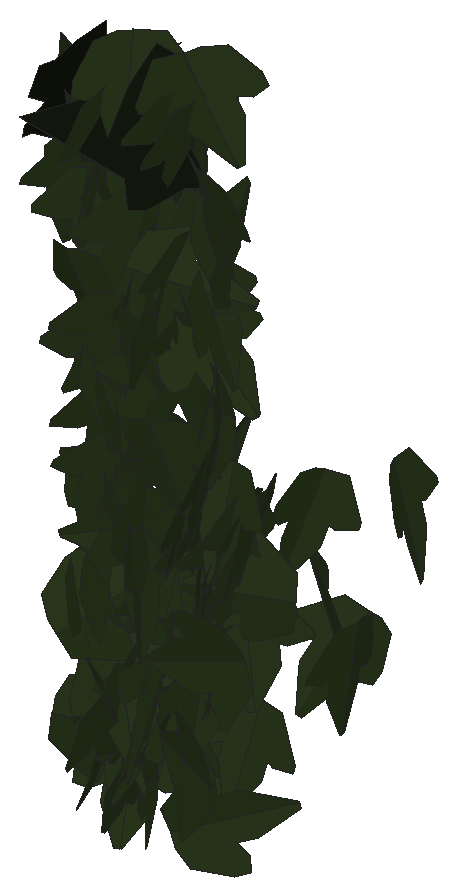
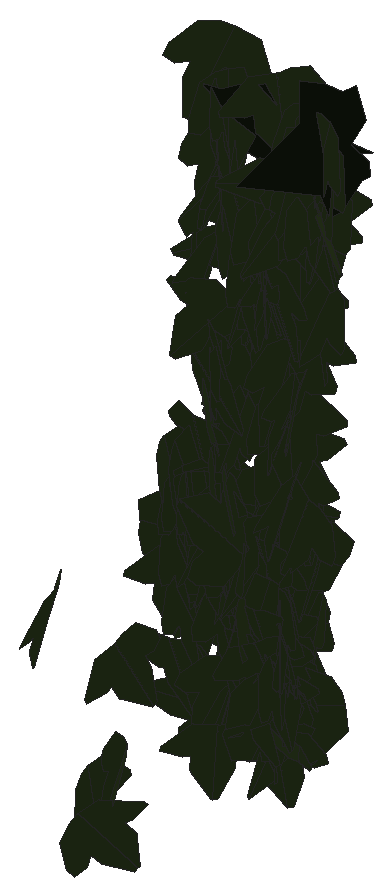
# SketchUp Ruby script. Lengths in inches.
U = 1.inch
M = Sketchup.active_model
def pt(a) = Geom::Point3d.new(a.map { |v| v * U })
def face(e, loops, mat)
  f = e.add_face(loops[0].map { |a| pt(a) })
  loops[1..].each { |l| e.add_face(l.map { |a| pt(a) }).erase! }
  f.material = f.back_material = mat if mat
  f
end
# faces: each face lists its corners as indices into pts; further lists are holes
def faces(e, pts, list, mat = nil) = list.each { |f| face(e, (f[0].is_a?(Array) ? f : [f]).map { |l| l.map { |i| pts[i] } }, mat) }
# xy, xz, yz: faces in a plane at the given z, y or x. An outline is a flat list of corners, or four numbers for a rectangle; further outlines are holes
def ring(l) = l.size == 4 ? [[l[0], l[1]], [l[2], l[1]], [l[2], l[3]], [l[0], l[3]]] : l.each_slice(2).to_a
def flat(e, list, mat, &to3) = list.each { |f| face(e, (f[0].is_a?(Array) ? f : [f]).map { |l| ring(l).map { |u, v| to3.(u, v) } }, mat) }
def xy(e, z, list, mat = nil) = flat(e, list, mat) { |x, y| [x, y, z] }
def xz(e, y, list, mat = nil) = flat(e, list, mat) { |x, z| [x, y, z] }
def yz(e, x, list, mat = nil) = flat(e, list, mat) { |y, z| [x, y, z] }
def lines(e, pts, list) = list.each { |a, b| e.add_line(pt(pts[a]), pt(pts[b])) }
# prism: a flat outline (further loops are holes) pulled along v
def prism(e, loops, v, mat = nil)
  f = face(e, loops, mat); d = Geom::Vector3d.new(v.map { |x| x * U })
  f.pushpull(f.normal.samedirection?(d) ? d.length : -d.length)
end
def box(e, o, s, mat = nil) = prism(e, [[o, [o[0] + s[0], o[1], o[2]], [o[0] + s[0], o[1] + s[1], o[2]], [o[0], o[1] + s[1], o[2]]]], [0, 0, s[2]], mat)
def at(x, y, z, deg = 0) = Geom::Transformation.translation(pt([x, y, z])) * Geom::Transformation.rotation(ORIGIN, Z_AXIS, deg.degrees)
def axes(o, x, y, z) = Geom::Transformation.new([*x, 0, *y, 0, *z, 0, *pt(o).to_a, 1])
def part(name) = M.definitions.add(name)
# library, detail: a bought-in or finely detailed component or shape, given as its bounding box
def library(name, o, s) = part(name).tap { |d| box(d.entities, o, s) }
def detail(e, o, s) = box(e.add_group.entities, o, s)
def put(e, d, t, mat = nil) = e.add_instance(d, t).tap { |i| i.material = mat if mat }
def group(e, t, mat = nil) = e.add_group.tap { |g| g.transformation = t; g.material = mat if mat }.entities
root = M.entities
M.materials.add("efeu1").color = [18, 25, 13]
M.materials.add("efeu2").color = [43, 57, 29]
c1 = part("ivyleaf_10")
p = [[0,0.5,-0.03],[-0.0625,2.02,-0.43],[-0.19,2.01,-0.46],[-0.54,1.05,-0.29],[-0.52,0.625,-0.18],[-0.83,0.76,-0.28],
  [-1.16,0.64,-0.33],[-1.15,0.33,-0.24],[-0.77,-0.39,0.02],[-0.3,-0.51,0.16],[0.04,-0.48,0.23],[-0.02,2.01,-0.4375],
  [-0.06,2.01,-0.43],[0.04,-0.49,0.23],[0.67,-0.49,0.14],[1.38,0.36,-0.2],[1.375,0.51,-0.24],[0.81,0.65,-0.19],
  [0.62,0.59,-0.15],[0.6,1.09,-0.28],[0.5,1.23,-0.31]]
faces(c1.entities,p,[[0,1,2,3,4,5,6,7,8,9,10],[11,12,0,13,14,15,16,17,18,19,20]],"efeu2")
c2 = part("ivyleaf_9")
p = [[1.54,2.16,1.25],[1.36,2.04,1.19],[-0.21,0.99,0.68],[-0.71,1.11,0.82],[-0.85,0.86,0.67],[-0.8,0.17,0.21],
  [-0.9,-0.01,0.1],[-0.67,-0.16,-0.02],[-0.08,-0.08,-0.05],[-0.03,-0.6,-0.4],[0.65,-0.88,-0.66],[0.83,-0.6,-0.49],
  [1.29,-0.42,-0.43],[1.8125,-0.07,-0.26],[1.21,0.44,0.15]]
faces(c2.entities,p,[[0,1,2,3,4,5,6,7,8,9,10,11,12,13,14]],"efeu1")
put(root,c1,axes([521.63,138.375,173.66],[0.03642,-0.63597,0.0421],[0.01639,-0.04122,-0.63686],[0.63715,0.03741,0.01397]))
put(root,c1,axes([521.68,137.33,181.72],[-0.16201,-0.67993,0.11129],[0.00026,-0.11439,-0.69846],[0.68898,-0.15984,0.02643]))
put(root,c1,axes([521.59,137.31,183],[-0.63085,0.3128,-0.09955],[0.04645,-0.12842,-0.69791],[-0.32495,-0.62562,0.09349]))
put(root,c1,axes([521.7,137.19,181.875],[-0.58468,0.38831,0.11251],[-0.11108,0.0359,-0.70119],[-0.38872,-0.59433,0.03116]))
put(root,c1,axes([521.73,137.81,173.7],[0.04033,-0.60534,-0.30444],[-0.00149,0.3049,-0.60645],[0.67758,0.0367,0.01678]))
put(root,c1,axes([521.33,137.39,181.05],[0.34543,-0.39762,-0.46848],[0.32054,-0.34191,0.52654],[-0.52424,-0.47106,0.01326]))
put(root,c2,axes([521.49,136.8,182.72],[0.24079,0.34365,0.64076],[0.3954,0.50457,-0.41919],[-0.61019,0.46256,-0.01878]))
put(root,c1,axes([521.68,138.15,174.76],[0.45192,-0.45158,-0.15955],[0.02127,0.23808,-0.61358],[0.47847,0.41594,0.17798]))
put(root,c1,axes([521.73,137.08,182.4375],[-0.65958,0.28506,-0.00532],[0.00194,-0.00894,-0.71851],[-0.28511,-0.65954,0.00744]))
put(root,c1,axes([521.42,137.88,176.49],[0.59836,-0.14425,0.27817],[0.30389,0.12093,-0.59097],[0.07641,0.64868,0.17203]))
put(root,c1,axes([521.66,138.17,174.29],[0.41426,-0.50056,0.10032],[0.10441,-0.04339,-0.64765],[0.49972,0.42402,0.05216]))
put(root,c1,axes([521.6875,137.17,180],[-0.63481,0.21978,-0.15697],[0.14667,-0.05616,-0.67176],[-0.22678,-0.65151,0.00495]))
put(root,c1,axes([522.03,137.49,176.72],[-0.62326,-0.0477,0.26578],[-0.26115,-0.0635,-0.6238],[0.06865,-0.67458,0.03993]))
put(root,c1,axes([521.92,138.41,173.25],[-0.3203,-0.53428,0.14995],[-0.00408,-0.17086,-0.61751],[0.55491,-0.30965,0.082]))
put(root,c1,axes([521.67,137.84,172.2],[-0.08853,-0.45137,-0.44245],[0.13261,-0.45009,0.43263],[-0.61799,-0.03192,0.15622]))
put(root,c1,axes([521.64,137.39,181.92],[-0.37113,-0.35946,-0.48251],[0.37331,0.30704,-0.51587],[0.47187,-0.52562,0.02863]))
put(root,c1,axes([521.93,138.38,172.29],[0.24532,0.56679,0.17941],[-0.06142,-0.16889,0.61752],[0.59133,-0.25268,-0.0103]))
put(root,c1,axes([521.98,136.99,174.07],[-0.51698,0.35185,0.17256],[-0.13825,0.10353,-0.62531],[-0.36668,-0.5351,-0.00752]))
put(root,c1,axes([521.83,137.77,178.42],[-0.43298,0.49382,-0.19017],[0.0645,-0.19463,-0.65226],[-0.52522,-0.43099,0.07667]))
put(root,c1,axes([521.4,137.54,172.83],[-0.12186,-0.03802,-0.69789],[0.68926,0.11084,-0.12639],[0.1158,-0.69972,0.0179]))
put(root,c1,axes([521.85,137.09,175.36],[-0.12313,0.68542,0.03123],[-0.0099,0.02995,-0.69638],[-0.68606,-0.12345,0.00444]))
put(root,c1,axes([522.04,137.58,177.97],[-0.34,-0.5928,0.00312],[-0.01009,0.0022,-0.68331],[0.59272,-0.34,-0.00985]))
put(root,c1,axes([521.95,138.38,173.95],[0.50097,0.35528,-0.1951],[-0.15047,-0.125,-0.614],[-0.37636,0.52288,-0.01422]))
put(root,c1,axes([521.88,138.03,172.17],[0.57312,0.28141,-0.0286],[-0.0251,-0.01377,-0.63848],[-0.28174,0.57366,-0.00129]))
put(root,c1,axes([521.9,137.78,176.71],[-0.18245,0.65594,0.01519],[0.0107,0.01874,-0.68067],[-0.65603,-0.18212,-0.01533]))
put(root,c1,axes([522.03,138.22,174.35],[0.60863,-0.1362,-0.15762],[-0.13614,0.10836,-0.61931],[0.15767,0.6193,0.0737]))
put(root,c1,axes([522.15,137.48,177.14],[-0.26854,-0.56151,0.25077],[-0.06831,-0.24471,-0.62109],[0.61116,-0.27407,0.04077]))
put(root,c1,axes([522.04,137.43,178.32],[-0.19363,0.62062,0.25663],[-0.09885,0.23784,-0.64975],[-0.66427,-0.2163,0.02188]))
put(root,c1,axes([521.99,137.36,181.68],[-0.02174,-0.32316,-0.72112],[0.15706,0.70523,-0.32077],[0.77445,-0.1521,0.04481]))
put(root,c1,axes([522.08,137.24,181.32],[-0.5316,-0.47405,0.02236],[0.08346,-0.12644,-0.69633],[0.46718,-0.51683,0.14984]))
put(root,c1,axes([522.2,137.12,179.11],[-0.61368,-0.27764,0.07523],[-0.03254,-0.10912,-0.66812],[0.28581,-0.60857,0.08547]))
put(root,c1,axes([522.12,137.625,172.21],[-0.02606,-0.38595,-0.51186],[0.04871,0.50961,-0.38673],[0.63921,-0.05457,0.0086]))
put(root,c1,axes([522.07,137.51,178.86],[-0.26527,-0.5787,-0.25013],[0.15361,0.20386,-0.63456],[0.61144,-0.30228,0.0509]))
put(root,c1,axes([522.3,142.29,172.375],[-0.32073,-0.37581,0.43332],[-0.02427,-0.48712,-0.44044],[0.57307,-0.23096,0.22386]))
put(root,c1,axes([522.25,138.17,172.9],[-0.19878,0.22652,0.58226],[0.02919,-0.60699,0.2461],[0.62408,0.10054,0.17395]))
put(root,c1,axes([522.22,138.06,174.73],[-0.65389,0.00582,-0.06624],[0.06629,0.00603,-0.65389],[-0.00518,-0.65721,-0.00659]))
put(root,c1,axes([521.8,137.38,182.13],[-0.01198,-0.03667,0.70751],[0.48021,0.51984,0.03507],[-0.52088,0.48009,0.01606]))
put(root,c1,axes([522.26,137,182.88],[-0.02378,-0.65358,-0.27372],[0.06735,0.27055,-0.65186],[0.70537,-0.04786,0.05301]))
put(root,c1,axes([522.22,141.71,173.38],[-0.44013,0.46308,-0.00992],[0.00995,-0.00423,-0.63886],[-0.46308,-0.44023,-0.00429]))
put(root,c1,axes([522.25,136.91,175.63],[-0.10043,0.55451,0.38958],[-0.09847,0.37772,-0.56301],[-0.67049,-0.13853,0.02433]))
put(root,c1,axes([522.7,137.67,176.16],[0.09478,0.07272,-0.66694],[-0.62373,-0.23852,-0.11465],[-0.24708,0.63,0.03358]))
put(root,c1,axes([522.03,137.92,173.1],[0.5933,0.06495,0.23202],[0.23022,0.02907,-0.59684],[-0.07106,0.63639,0.00358]))
put(root,c1,axes([522.24,137.56,173.14],[0.62736,-0.16316,0.01158],[0.01079,-0.00451,-0.64823],[0.16322,0.62745,-0.00165]))
put(root,c1,axes([522.36,137.55,180.3],[0.59763,-0.33867,-0.11277],[-0.08526,0.07812,-0.68645],[0.34662,0.60314,0.02559]))
put(root,c1,axes([521.99,136.75,174.92],[0.25969,0.18711,-0.62084],[0.47918,0.39519,0.31954],[0.43686,-0.5447,0.01857]))
put(root,c1,axes([522.55,137.71,173.72],[-0.31838,-0.45924,0.38935],[-0.14092,-0.37136,-0.55326],[0.58535,-0.33919,0.07858]))
put(root,c1,axes([522.4,138.08,174.41],[0.14583,-0.6453,0.03566],[0.01217,-0.03381,-0.66156],[0.64617,0.14627,0.00441]))
put(root,c1,axes([522.35,137.78,175.39],[0.64915,-0.12838,-0.01838],[-0.01786,0.00443,-0.66172],[0.12846,0.64939,0.00088]))
put(root,c1,axes([522.05,138.29,173.7],[0.50446,0.05953,0.40313],[0.39466,0.08844,-0.50692],[-0.10151,0.63967,0.03257]))
put(root,c1,axes([522.45,136.71,173.73],[-0.00167,-0.56962,-0.38031],[0.05497,0.37898,-0.56786],[0.68271,-0.03191,0.04479]))
put(root,c1,axes([522.53,137.49,175.3125],[-0.1041,0.25061,0.68665],[-0.23782,0.64422,-0.27118],[-0.69118,-0.25941,-0.01011]))
put(root,c1,axes([522.51,141.26,175.02],[0.13889,0.55426,-0.30055],[-0.2022,-0.25234,-0.5588],[-0.5972,0.21434,0.1193]))
put(root,c1,axes([522.66,137.42,172.43],[0.35384,-0.33254,-0.46485],[-0.24805,0.4032,-0.47725],[0.51491,0.42275,0.08952]))
put(root,c1,axes([522.59,136.98,179.76],[-0.47977,-0.51467,0.0466],[-0.02902,-0.03666,-0.7036],[0.51596,-0.48064,0.00376]))
put(root,c1,axes([522.35,137.19,174.12],[0.35154,0.60451,0.06889],[0.03476,0.05947,-0.69929],[-0.60743,0.35326,-0.00015]))
put(root,c1,axes([522.64,137.61,173.77],[-0.14546,-0.55469,0.3004],[-0.07034,-0.2921,-0.57342],[0.62687,-0.16148,0.00536]))
put(root,c1,axes([522.41,138.93,172.51],[0.44756,0.45412,0.03932],[0.02997,0.02566,-0.63759],[-0.45483,0.44855,-0.00332]))
put(root,c1,axes([522.51,138.54,175.83],[0.18284,-0.60012,0.45518],[-0.07852,0.45066,0.6257],[-0.74911,-0.19371,0.04552]))
put(root,c1,axes([522.7,138.1,174.45],[-0.46111,-0.44904,0.0508],[-0.03478,-0.0371,-0.64363],[0.45057,-0.46242,0.0023]))
put(root,c1,axes([522.5625,137.17,183.56],[0.43145,0.56179,-0.0689],[-0.09208,-0.01581,-0.70553],[-0.55845,0.43663,0.0631]))
put(root,c1,axes([523.04,136.75,176.61],[-0.25387,0.29947,0.56995],[-0.57888,0.162,-0.34297],[-0.28182,-0.60253,0.19106]))
put(root,c1,axes([522.71,137.23,181.21],[-0.29708,-0.63648,0.12707],[0.00882,-0.1437,-0.69913],[0.64898,-0.2894,0.06768]))
put(root,c1,axes([522.68,137.37,180.69],[0.28487,-0.61924,-0.18683],[0.00222,0.20508,-0.67635],[0.64681,0.27203,0.08461]))
put(root,c1,axes([522.71,138.05,175.41],[0.47458,0.44296,-0.12521],[-0.20774,0.04562,-0.626],[-0.41077,0.48869,0.17193]))
put(root,c1,axes([522.61,138.01,173.27],[0.09617,-0.31245,0.57498],[0.15588,-0.55349,-0.32685],[0.63556,0.18304,-0.00684]))
put(root,c1,axes([523.03,138.06,175.6],[-0.46684,-0.27826,0.38278],[-0.33015,-0.19373,-0.54347],[0.33905,-0.57178,-0.00214]))
put(root,c1,axes([522.81,137.88,175.24],[-0.2087,-0.61594,0.02172],[-0.01243,-0.01872,-0.65031],[0.6162,-0.20899,-0.00576]))
put(root,c1,axes([522.81,138.06,175.62],[-0.01373,-0.66369,0.00154],[-0.00088,-0.00152,-0.66383],[0.66369,-0.01373,-0.00085]))
put(root,c1,axes([522.78,138.16,175.42],[-0.56831,0.31824,0.01332],[-0.00761,0.01367,-0.6513],[-0.31843,-0.5683,-0.00821]))
put(root,c1,axes([522.98,137.48,178.76],[-0.38059,-0.496,0.29972],[-0.13193,-0.27501,-0.62262],[0.56431,-0.39881,0.05658]))
put(root,c2,axes([523.43,137.14,182.625],[-0.49023,0.07444,0.60663],[-0.6038,0.0615,-0.49549],[-0.09469,-0.77753,0.01889]))
put(root,c1,axes([522.89,137.27,180.31],[-0.62337,0.28816,0.08014],[-0.07367,0.03162,-0.68674],[-0.28988,-0.6277,0.0022]))
put(root,c1,axes([522.6875,138.27,173.19],[-0.53678,-0.26976,-0.24742],[0.26869,0.00785,-0.59149],[0.24858,-0.591,0.10507]))
put(root,c1,axes([522.81,141.6,172.66],[0.05917,-0.65084,0.09162],[0.1185,-0.07991,-0.64425],[0.64648,0.07422,0.1097]))
put(root,c1,axes([522.86,137.15,179.79],[0.44935,-0.52861,-0.02147],[-0.01313,0.01702,-0.69379],[0.52888,0.44954,0.00101]))
put(root,c1,axes([522.87,136.91,179.95],[-0.17162,0.65159,0.18226],[-0.08869,0.16474,-0.67248],[-0.67076,-0.18849,0.04229]))
put(root,c1,axes([522.95,137.4,180.33],[-0.01495,-0.6986,-0.082],[-0.00965,0.08221,-0.69867],[0.70333,-0.01372,-0.01133]))
put(root,c1,axes([522.87,137.99,174.18],[-0.42597,0.49059,-0.00356],[0.00271,-0.00236,-0.64972],[-0.4906,-0.42598,-0.0005]))
put(root,c1,axes([522.76,137.1875,176.06],[-0.12781,0.65961,-0.33241],[0.07087,-0.32484,-0.67184],[-0.73523,-0.14598,-0.00698]))
put(root,c1,axes([522.9,137.94,176.5],[0.28683,-0.60631,0.02491],[0.03244,-0.0122,-0.6703],[0.60596,0.28766,0.02409]))
put(root,c1,axes([522.98,138.01,176.19],[-0.32108,-0.58141,0.05639],[0.02075,-0.07566,-0.66194],[0.58377,-0.3171,0.05454]))
put(root,c1,axes([523.01,138.1875,175.39],[-0.18352,-0.62046,0.05668],[-0.01267,-0.05536,-0.64702],[0.62292,-0.18392,0.00354]))
put(root,c1,axes([522.875,138.12,172.79],[-0.18715,0.61657,-0.03597],[0.01313,-0.03361,-0.64434],[-0.61748,-0.18758,-0.0028]))
put(root,c1,axes([522.96,137.1,173.95],[0.47676,-0.48267,0.05189],[0.02765,-0.04561,-0.67832],[0.48466,0.47741,-0.01234]))
put(root,c1,axes([523,137.69,177.73],[-0.5957,0.31932,-0.04803],[0.05183,-0.00492,-0.67559],[-0.31873,-0.59762,-0.0201]))
put(root,c1,axes([523.02,137.2,177.84],[-0.65366,-0.13361,-0.11217],[0.10788,0.03226,-0.6671],[0.13709,-0.66243,-0.00987]))
put(root,c1,axes([523.01,138.1,175.23],[-0.15471,-0.62445,0.09323],[0.16042,-0.13171,-0.61602],[0.61065,-0.1236,0.18545]))
put(root,c1,axes([523.18,137.42,181.46],[0.67248,0.02095,-0.20491],[-0.20306,0.18461,-0.64756],[0.03449,0.67833,0.18256]))
put(root,c1,axes([523.17,136.8125,180.01],[0.09958,-0.45863,-0.5924],[0.03202,0.59967,-0.45888],[0.7485,0.03536,0.09845]))
put(root,c1,axes([523.07,138.19,175.42],[-0.16099,0.49685,-0.39518],[0.03221,-0.40077,-0.517],[-0.63403,-0.14652,0.07407]))
put(root,c1,axes([523.39,138.05,176.25],[-0.61445,-0.01059,0.22603],[-0.22307,-0.08152,-0.61021],[0.03801,-0.64961,0.0729]))
put(root,c1,axes([523.0625,138.21,175.4],[0.40691,-0.46645,0.21414],[0.16156,-0.14297,-0.61844],[0.48717,0.43702,0.02623]))
put(root,c1,axes([523.26,137.86,176.65],[0.23845,-0.62034,-0.12543],[-0.00969,0.13044,-0.66356],[0.63282,0.23575,0.03711]))
put(root,c1,axes([523.18,138.24,175.49],[-0.20706,0.62099,-0.0177],[0.00474,-0.01707,-0.6546],[-0.62122,-0.20712,0.0009]))
put(root,c1,axes([523.71,137.6,178.3],[0.20838,-0.14312,-0.74198],[-0.54771,0.50165,-0.25058],[0.52059,0.58507,0.03336]))
put(root,c1,axes([523.35,137.35,180.84],[0.12518,-0.69334,0.05727],[0.02068,-0.05446,-0.70447],[0.69539,0.12643,0.01064]))
put(root,c1,axes([523.52,138.21,174.47],[-0.12228,-0.64274,-0.0049],[0.00537,0.00397,-0.65425],[0.64273,-0.12232,0.00453]))
put(root,c1,axes([523.39,137.75,175.41],[0.40901,-0.48828,0.13906],[0.07859,-0.11552,-0.63681],[0.50157,0.41627,-0.01362]))
put(root,c1,axes([523.54,137.21,183.15],[-0.26807,-0.65992,-0.06819],[0.02276,0.06435,-0.71228],[0.66304,-0.26902,-0.00312]))
put(root,c1,axes([523.47,137.62,174.18],[0.1228,0.61212,-0.19031],[-0.09599,-0.17402,-0.62168],[-0.63379,0.14495,0.05729]))
put(root,c1,axes([523.6,138.15,176.21],[-0.15045,-0.63945,-0.04545],[-0.00104,0.04693,-0.6568],[0.64106,-0.15,-0.01173]))
put(root,c1,axes([523.6,138.14,176.19],[0.14697,-0.62286,-0.15731],[-0.00279,0.16075,-0.63911],[0.64241,0.1432,0.03321]))
put(root,c1,axes([523.6,137.55,178.83],[0.42917,-0.52205,-0.12273],[-0.05088,0.11685,-0.67494],[0.53387,0.43081,0.03434]))
put(root,c1,axes([523.67,138.13,176.29],[-0.05495,-0.65616,-0.02433],[-0.01212,0.02543,-0.65831],[0.6565,-0.05445,-0.01419]))
put(root,c1,axes([523.16,136.9,180.57],[-0.18407,-0.14395,-0.67044],[0.63552,0.22489,-0.22277],[0.25752,-0.65787,0.07055]))
put(root,c1,axes([523.67,138.21,175.36],[-0.05126,-0.65201,0.02266],[0.00081,-0.02279,-0.65402],[0.65241,-0.0512,0.0026]))
put(root,c1,axes([523.65,137.07,183.07],[0.07618,-0.70911,-0.035],[0.01535,0.03684,-0.71293],[0.7098,0.07531,0.01917]))
put(root,c1,axes([523.64,137.63,174.51],[0.44465,-0.4996,-0.08924],[-0.04353,0.08067,-0.66848],[0.50564,0.44628,0.02093]))
put(root,c1,axes([524.05,136.72,173.16],[0.05453,-0.07883,-0.71109],[-0.50834,0.49756,-0.09414],[0.50344,0.51094,-0.01803]))
put(root,c1,axes([523.69,137.45,177.66],[0.26032,-0.64141,-0.04392],[-0.01503,0.0413,-0.69222],[0.64274,0.26075,0.0016]))
put(root,c1,axes([523.34,137.59,179.43],[0.4578,0.2454,0.46092],[0.39447,0.23911,-0.51911],[-0.34214,0.60404,0.01823]))
put(root,c1,axes([524.22,138.17,175.38],[-0.01493,0.03366,0.65514],[-0.57318,-0.3194,0.00335],[0.31907,-0.5722,0.03667]))
put(root,c1,axes([524.09,136.95,181.98],[-0.42614,0.38818,0.4143],[-0.41119,0.14618,-0.55989],[-0.39148,-0.57608,0.1371]))
put(root,c1,axes([523.9,137.12,182.07],[-0.64863,0.26015,0.1042],[-0.08908,0.05768,-0.69857],[-0.26571,-0.65441,-0.02015]))
put(root,c1,axes([523.78,138.23,173.27],[0.64976,-0.01512,-0.06124],[-0.06095,0.01261,-0.64984],[0.01623,0.65251,0.01114]))
put(root,c1,axes([523.75,138.13,174.86],[0.46998,0.44734,0.08411],[-0.00023,0.12113,-0.64296],[-0.45518,0.46182,0.08716]))
put(root,c1,axes([523.76,137.69,177.14],[0.65356,-0.13508,0.0773],[0.07324,-0.0275,-0.66727],[0.13732,0.65754,-0.01202]))
put(root,c1,axes([524.03,137.13,178.45],[0.31653,-0.53759,-0.39212],[-0.12572,0.37809,-0.61983],[0.65342,0.33316,0.07069]))
put(root,c1,axes([523.88,137.9375,176.65],[0.12732,-0.63004,0.19354],[0.10071,-0.1762,-0.63986],[0.65135,0.1504,0.0611]))
put(root,c1,axes([523.84,137.28,180.29],[-0.12402,0.68197,0.07052],[0.00244,0.0721,-0.69298],[-0.6856,-0.12311,-0.01522]))
put(root,c1,axes([523.55,137.35,171.92],[-0.1617,-0.16716,0.65401],[0.41703,0.50409,0.23194],[-0.53081,0.44696,-0.017]))
put(root,c1,axes([524.07,137.04,181.01],[0.08405,0.2002,-0.74136],[-0.09276,0.74297,0.19012],[0.76229,0.06834,0.10488]))
put(root,c1,axes([524.375,136.86,175.01],[0.27639,0.02308,-0.64568],[-0.61862,0.21208,-0.25722],[0.18641,0.66956,0.10373]))
put(root,c1,axes([524,138.1,176.73],[0.1343,-0.64736,-0.00691],[-0.01298,0.00436,-0.66104],[0.64726,0.13441,-0.01182]))
put(root,c1,axes([523.81,137.01,183.82],[-0.59422,-0.32991,-0.26224],[0.30148,-0.01601,-0.66299],[0.29448,-0.64931,0.14959]))
put(root,c1,axes([523.86,141.41,175.58],[-0.21981,0.63903,-0.06258],[0.03354,-0.05463,-0.67563],[-0.64121,-0.22192,-0.01389]))
